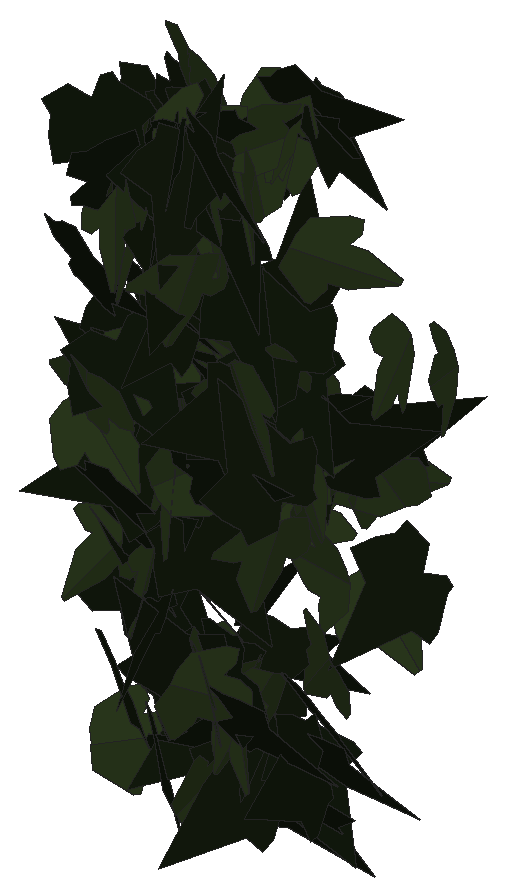
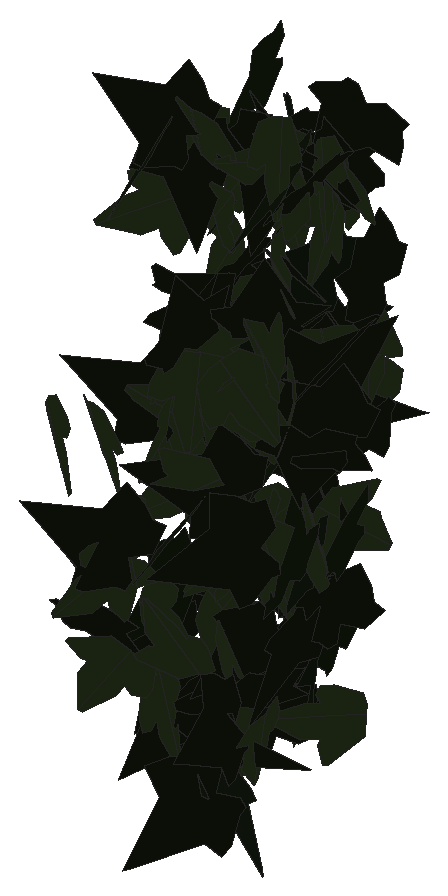
# SketchUp Ruby script. Lengths in inches.
U = 1.inch
M = Sketchup.active_model
def pt(a) = Geom::Point3d.new(a.map { |v| v * U })
def face(e, loops, mat)
  f = e.add_face(loops[0].map { |a| pt(a) })
  loops[1..].each { |l| e.add_face(l.map { |a| pt(a) }).erase! }
  f.material = f.back_material = mat if mat
  f
end
# faces: each face lists its corners as indices into pts; further lists are holes
def faces(e, pts, list, mat = nil) = list.each { |f| face(e, (f[0].is_a?(Array) ? f : [f]).map { |l| l.map { |i| pts[i] } }, mat) }
# xy, xz, yz: faces in a plane at the given z, y or x. An outline is a flat list of corners, or four numbers for a rectangle; further outlines are holes
def ring(l) = l.size == 4 ? [[l[0], l[1]], [l[2], l[1]], [l[2], l[3]], [l[0], l[3]]] : l.each_slice(2).to_a
def flat(e, list, mat, &to3) = list.each { |f| face(e, (f[0].is_a?(Array) ? f : [f]).map { |l| ring(l).map { |u, v| to3.(u, v) } }, mat) }
def xy(e, z, list, mat = nil) = flat(e, list, mat) { |x, y| [x, y, z] }
def xz(e, y, list, mat = nil) = flat(e, list, mat) { |x, z| [x, y, z] }
def yz(e, x, list, mat = nil) = flat(e, list, mat) { |y, z| [x, y, z] }
def lines(e, pts, list) = list.each { |a, b| e.add_line(pt(pts[a]), pt(pts[b])) }
# prism: a flat outline (further loops are holes) pulled along v
def prism(e, loops, v, mat = nil)
  f = face(e, loops, mat); d = Geom::Vector3d.new(v.map { |x| x * U })
  f.pushpull(f.normal.samedirection?(d) ? d.length : -d.length)
end
def box(e, o, s, mat = nil) = prism(e, [[o, [o[0] + s[0], o[1], o[2]], [o[0] + s[0], o[1] + s[1], o[2]], [o[0], o[1] + s[1], o[2]]]], [0, 0, s[2]], mat)
def at(x, y, z, deg = 0) = Geom::Transformation.translation(pt([x, y, z])) * Geom::Transformation.rotation(ORIGIN, Z_AXIS, deg.degrees)
def axes(o, x, y, z) = Geom::Transformation.new([*x, 0, *y, 0, *z, 0, *pt(o).to_a, 1])
def part(name) = M.definitions.add(name)
# library, detail: a bought-in or finely detailed component or shape, given as its bounding box
def library(name, o, s) = part(name).tap { |d| box(d.entities, o, s) }
def detail(e, o, s) = box(e.add_group.entities, o, s)
def put(e, d, t, mat = nil) = e.add_instance(d, t).tap { |i| i.material = mat if mat }
def group(e, t, mat = nil) = e.add_group.tap { |g| g.transformation = t; g.material = mat if mat }.entities
root = M.entities
M.materials.add("efeu1").color = [18, 25, 13]
M.materials.add("efeu2").color = [43, 57, 29]
c1 = part("ivyleaf_9")
p = [[1.54,2.16,1.25],[1.36,2.04,1.19],[-0.21,0.99,0.68],[-0.71,1.11,0.82],[-0.85,0.86,0.67],[-0.8,0.17,0.21],
  [-0.9,-0.01,0.1],[-0.67,-0.16,-0.02],[-0.08,-0.08,-0.05],[-0.03,-0.6,-0.4],[0.65,-0.88,-0.66],[0.83,-0.6,-0.49],
  [1.29,-0.42,-0.43],[1.8125,-0.07,-0.26],[1.21,0.44,0.15]]
faces(c1.entities,p,[[0,1,2,3,4,5,6,7,8,9,10,11,12,13,14]],"efeu1")
c2 = part("ivyleaf_10")
p = [[0,0.5,-0.03],[-0.0625,2.02,-0.43],[-0.19,2.01,-0.46],[-0.54,1.05,-0.29],[-0.52,0.625,-0.18],[-0.83,0.76,-0.28],
  [-1.16,0.64,-0.33],[-1.15,0.33,-0.24],[-0.77,-0.39,0.02],[-0.3,-0.51,0.16],[0.04,-0.48,0.23],[-0.02,2.01,-0.4375],
  [-0.06,2.01,-0.43],[0.04,-0.49,0.23],[0.67,-0.49,0.14],[1.38,0.36,-0.2],[1.375,0.51,-0.24],[0.81,0.65,-0.19],
  [0.62,0.59,-0.15],[0.6,1.09,-0.28],[0.5,1.23,-0.31]]
faces(c2.entities,p,[[0,1,2,3,4,5,6,7,8,9,10],[11,12,0,13,14,15,16,17,18,19,20]],"efeu2")
put(root,c1,axes([35.11,223.37,217.44],[0.41887,-0.24066,-0.12894],[-0.10462,0.07663,-0.48289],[0.25219,0.43152,0.01384]))
put(root,c1,axes([35.23,224.11,218.95],[-0.24521,-0.33335,-0.28062],[0.17028,0.22309,-0.4138],[0.40109,-0.29851,0.00412]))
put(root,c1,axes([34.97,223.83,218.99],[0.11939,-0.07912,0.47905],[0.46236,-0.13208,-0.13704],[0.14823,0.47571,0.04163]))
put(root,c2,axes([35.53,223.26,217.38],[-0.13067,-0.26306,0.40463],[-0.05565,-0.40819,-0.28335],[0.4794,-0.11909,0.0774]))
put(root,c1,axes([35.2,223.61,216.17],[-0.13742,0.01876,0.48038],[0.47886,-0.03889,0.13851],[0.04256,0.49813,-0.00728]))
put(root,c1,axes([35.72,225.29,214.58],[-0.26797,0.41954,0.04669],[-0.02794,0.03755,-0.4978],[-0.4212,-0.2694,0.00332]))
put(root,c2,axes([35.38,223.7,216.95],[0.28986,-0.40739,-0.00394],[0.00449,-0.00164,0.49998],[-0.40739,-0.28988,0.00271]))
put(root,c1,axes([35.42,224,216.1875],[0.14476,-0.23263,-0.41824],[-0.21797,0.35696,-0.27398],[0.42607,0.26165,0.00194]))
put(root,c1,axes([35.08,222.9,220.77],[0.24977,-0.19631,0.38611],[0.29109,-0.25397,-0.31743],[0.32075,0.38335,-0.01258]))
put(root,c2,axes([35.42,224.85,215.12],[-0.04426,0.49201,-0.07725],[0.00837,-0.07681,-0.49399],[-0.49797,-0.04502,-0.00144]))
put(root,c1,axes([35.5,225.33,215.32],[0.06139,0.22899,0.44022],[0.13132,0.42027,-0.23692],[-0.47853,0.14471,-0.00854]))
put(root,c1,axes([35.3,223.6,219.8125],[0.06581,-0.4799,0.12394],[0.03016,-0.12092,-0.48422],[0.49473,0.07121,0.01303]))
put(root,c1,axes([35.33,225.94,214.64],[0.41277,0.24469,0.14052],[0.12007,0.07302,-0.47985],[-0.25535,0.42988,0.00152]))
put(root,c2,axes([35.27,223.34,214.64],[0.05743,-0.04345,-0.49479],[0.41152,0.28306,0.02291],[0.27812,-0.40986,0.06827]))
put(root,c2,axes([35.71,222.39,219.64],[-0.48065,0.03711,0.13265],[-0.13227,0.01008,-0.48208],[-0.03845,-0.49852,0.00013]))
put(root,c1,axes([35.8,223.35,219.15],[0.10877,0.02796,0.48722],[-0.48134,-0.07619,0.11183],[0.0805,-0.49337,0.01035]))
put(root,c2,axes([35.58,223.28,221.6875],[-0.42485,0.26195,-0.02976],[0.02473,-0.0166,-0.49911],[-0.26247,-0.42557,0.00115]))
put(root,c1,axes([35.42,223.96,222.47],[0.04736,-0.49619,0.03945],[0.01761,-0.03793,-0.49825],[0.49744,0.04858,0.01388]))
put(root,c1,axes([35.375,225.01,217.75],[0.28746,0.18449,0.36514],[0.3003,0.20791,-0.34146],[-0.27782,0.41562,0.00872]))
put(root,c1,axes([35.36,224.36,217.07],[0.37616,-0.19146,-0.26804],[0.24095,-0.11749,0.42206],[-0.22461,-0.4467,0.00388]))
put(root,c2,axes([35.82,224.03,223.04],[-0.43216,0.1415,0.20788],[-0.19349,0.07688,-0.45459],[-0.16062,-0.47336,-0.01169]))
put(root,c2,axes([35.72,223.19,222.4],[0.1112,-0.45507,-0.17477],[-0.02862,0.17286,-0.4683],[0.48664,0.11415,0.0124]))
put(root,c2,axes([35.69,224.3125,217.26],[0.08688,-0.47772,0.11932],[0.0325,-0.11533,-0.48543],[0.49132,0.0921,0.01101]))
put(root,c1,axes([36.13,225.24,214.84],[-0.36335,-0.01145,0.34328],[-0.34323,-0.00665,-0.36352],[0.01289,-0.49982,-0.00303]))
put(root,c2,axes([36.09,223.96,218.9],[0.05965,0.00155,-0.49643],[-0.47281,-0.15222,-0.05728],[-0.1513,0.47626,-0.0167]))
put(root,c2,axes([35.44,224.55,220.08],[-0.10964,0.0224,0.48732],[0.46723,-0.1388,0.1115],[0.14028,0.47982,0.0095]))
put(root,c1,axes([35.61,223.96,222.66],[0.38029,-0.24282,-0.21546],[-0.14822,0.16536,-0.44798],[0.28881,0.40459,0.05379]))
put(root,c1,axes([35.53,222.66,222.99],[-0.15015,-0.16353,-0.44801],[0.32706,0.30654,-0.22151],[0.34711,-0.35957,0.01491]))
put(root,c2,axes([35.61,224.03,219.35],[-0.15125,0.28226,-0.38399],[0.17892,-0.33977,-0.32023],[-0.44171,-0.23428,0.00178]))
put(root,c1,axes([35.56,223.13,215.52],[0.02902,-0.19959,0.45752],[0.15002,-0.43361,-0.19868],[0.47608,0.1488,0.03472]))
put(root,c2,axes([35.77,223.15,219.76],[0.38168,0.31827,-0.055],[-0.04252,-0.0349,-0.49697],[-0.32018,0.38404,0.00043]))
put(root,c2,axes([36.07,224.64,219.76],[-0.30192,-0.25974,0.30229],[-0.21257,-0.21584,-0.39777],[0.33713,-0.36871,0.01991]))
put(root,c1,axes([36.11,222.93,218.58],[-0.07723,-0.19879,-0.45224],[-0.10899,-0.43959,0.21185],[-0.48183,0.1313,0.02457]))
put(root,c2,axes([35.61,222.46,219.2],[0.33561,0.22296,0.29606],[0.25085,0.15738,-0.40287],[-0.27284,0.41895,-0.00622]))
put(root,c1,axes([35.74,222.33,218.55],[0.48148,0.07307,-0.11331],[-0.11189,-0.01795,-0.48699],[-0.07524,0.49431,-0.00093]))
put(root,c1,axes([35.54,223.8,216.97],[0.39706,-0.2638,0.15084],[0.12924,-0.07802,-0.47666],[0.27503,0.41752,0.00623]))
put(root,c2,axes([35.68,226.01,216.47],[0.44446,-0.00098,-0.22903],[0.22785,0.05266,0.44194],[0.02325,-0.49722,0.04726]))
put(root,c2,axes([36.09,224.58,219.41],[0.26444,0.21311,-0.36695],[-0.32739,-0.17262,-0.33618],[-0.26998,0.41807,0.04824]))
put(root,c1,axes([35.67,222.48,222.15],[0.25324,0.125,0.41261],[0.36552,0.1915,-0.28235],[-0.22862,0.44464,0.00561]))
put(root,c2,axes([35.78,222.65,221.89],[0.42237,-0.1762,0.20138],[0.19446,-0.05637,-0.45717],[0.18381,0.46452,0.02091]))
put(root,c1,axes([35.82,222.74,220.02],[-0.03193,-0.31942,-0.38334],[0.119,0.36817,-0.31669],[0.48458,-0.11146,0.05251]))
put(root,c2,axes([36.0625,224.56,217.26],[0.01299,0.04959,0.49737],[-0.10661,0.48636,-0.0457],[-0.48833,-0.10487,0.02321]))
put(root,c1,axes([36.25,224.1875,214.95],[-0.32221,-0.2956,0.24249],[-0.17196,-0.17119,-0.43718],[0.34148,-0.36512,0.00865]))
put(root,c1,axes([36.37,223.55,222.48],[-0.4892,-0.03288,0.09797],[-0.09709,-0.01611,-0.49022],[0.0354,-0.49866,0.00938]))
put(root,c1,axes([35.72,223.11,220.66],[0.32158,-0.23998,0.29832],[0.25134,-0.16156,-0.40091],[0.28881,0.40781,0.01672]))
put(root,c1,axes([35.97,224.25,218.03],[-0.01879,-0.36522,0.34097],[0.03743,-0.34129,-0.36349],[0.49824,0.01187,0.04016]))
put(root,c1,axes([35.93,223.4,214.48],[0.01277,-0.11607,0.48617],[0.09594,-0.47672,-0.11633],[0.49054,0.09626,0.0101]))
put(root,c1,axes([36.26,223.74,220.06],[-0.41795,-0.16121,0.2221],[0.21248,0.06603,0.44777],[-0.1737,0.46867,0.01332]))
put(root,c1,axes([35.9,223.02,217.26],[-0.06107,0.09764,0.48656],[0.29406,-0.38777,0.11472],[0.39975,0.30017,-0.01007]))
put(root,c2,axes([36.25,222.51,221.72],[0.30026,-0.39695,-0.04767],[-0.02885,0.03794,-0.49772],[0.39876,0.30164,-0.00012]))
put(root,c1,axes([36.24,223.46,222.58],[0.30048,0.38408,-0.11043],[-0.07085,-0.08478,-0.48764],[-0.39331,0.3087,0.00347]))
put(root,c2,axes([36.17,222.82,217.55],[0.35041,-0.34361,0.09561],[0.06886,-0.06634,-0.49077],[0.34996,0.35711,0.00083]))
put(root,c2,axes([35.89,223.625,222.09],[-0.1257,0.03507,-0.48267],[0.42294,-0.23442,-0.12718],[-0.23521,-0.44025,0.02926]))
put(root,c1,axes([36.02,223.84,214.39],[0.45386,0.19835,0.06833],[-0.0676,-0.0159,0.49515],[0.1986,-0.4587,0.01239]))
put(root,c1,axes([36.45,223.08,220.55],[-0.4907,0.07951,-0.05378],[0.05327,-0.00747,-0.4971],[-0.07986,-0.49358,-0.00114]))
put(root,c1,axes([35.9,224.79,218.24],[0.18575,0.00341,0.46421],[0.459,0.07338,-0.1842],[-0.06938,0.49457,0.02413]))
put(root,c2,axes([36.15,223.57,220.875],[0.26451,-0.28956,0.31014],[0.20161,-0.23581,-0.39211],[0.37334,0.33249,-0.00799]))
put(root,c2,axes([36.07,223.44,222.36],[0.06505,0.03302,-0.49465],[0.34012,0.35999,0.06876],[0.36067,-0.34543,0.02438]))
put(root,c1,axes([36.08,225.88,217.97],[0.10408,-0.46346,0.15613],[0.04191,-0.15059,-0.47494],[0.48725,0.11194,0.0075]))
put(root,c1,axes([36.34,222.9,217.11],[-0.34358,0.12262,-0.34193],[0.30736,-0.15271,-0.3636],[-0.19361,-0.46005,0.02956]))
put(root,c2,axes([36.3,223.88,214.26],[0.00266,0.14559,0.47833],[0.01517,0.47809,-0.1456],[-0.49976,0.01529,-0.00187]))
put(root,c1,axes([36.3,223.12,222.6],[-0.26525,0.05667,-0.42004],[0.39923,-0.13298,-0.27005],[-0.14232,-0.47865,0.02529]))
put(root,c1,axes([36.57,222.92,216.03],[0.26558,-0.04971,0.42071],[-0.4055,0.11391,0.26943],[-0.12263,-0.48431,0.02019]))
put(root,c1,axes([36.2,223.63,215.72],[-0.02949,-0.14551,-0.47745],[0.12947,0.45968,-0.1481],[0.48205,-0.13236,0.01056]))
put(root,c2,axes([36.81,225.16,215.31],[-0.31378,0.10324,0.37534],[-0.36425,0.09222,-0.32988],[-0.13735,-0.48045,0.01734]))
put(root,c1,axes([36.54,222.86,222.04],[-0.37488,0.30609,0.12561],[0.09597,-0.08107,0.48396],[0.31663,0.38696,0.00203]))
put(root,c2,axes([36.26,224.99,218.33],[0.13189,0.16552,0.453],[0.27203,0.36227,-0.21156],[-0.39826,0.30226,0.00551]))
put(root,c2,axes([36.86,225.18,216.42],[0.082,-0.04456,-0.49121],[-0.40511,0.27796,-0.09284],[0.28135,0.41322,0.00948]))
put(root,c2,axes([36.52,223.21,214.36],[0.05428,-0.2838,0.40806],[-0.02389,0.40852,0.2873],[-0.49647,-0.05069,0.0308]))
put(root,c2,axes([36.76,224.09,221.65],[0.35124,-0.08107,0.34649],[-0.32948,0.10983,0.3597],[-0.13444,-0.481,0.02373]))
put(root,c1,axes([36.45,222.91,221.26],[-0.00194,-0.41269,0.28228],[0.0149,-0.2822,-0.41248],[0.49977,0.00681,0.01339]))
put(root,c2,axes([36.67,223.89,215.65],[0.11441,-0.46423,0.14627],[0.03267,-0.1426,-0.47812],[0.48564,0.11896,-0.0023]))
put(root,c1,axes([36.61,223.11,222.39],[-0.16349,-0.47012,0.04754],[-0.01569,-0.04487,-0.49774],[0.47226,-0.16424,-0.00008]))
put(root,c1,axes([36.99,223.76,218.28],[-0.28282,0.37753,0.16578],[-0.10541,0.12815,-0.47166],[-0.39862,-0.30175,0.00711]))
put(root,c2,axes([36.47,222.8,218.71],[0.30008,-0.22495,0.33068],[0.27002,-0.19102,-0.37497],[0.29503,0.40362,0.00684]))
put(root,c1,axes([36.79,224.66,220.02],[-0.16671,-0.28768,0.37343],[0.22334,0.30061,0.33129],[-0.41512,0.27726,0.02826]))
put(root,c1,axes([36.36,223.78,219.17],[0.31325,-0.2476,0.30095],[0.24595,-0.17392,-0.39908],[0.3023,0.39806,0.01283]))
put(root,c2,axes([36.86,224.36,219.45],[-0.47399,-0.15791,0.02006],[-0.01831,-0.00852,-0.49959],[0.15812,-0.47433,0.00229]))
put(root,c2,axes([36.9375,222.57,221.42],[-0.20033,-0.44711,0.09983],[-0.03568,-0.0934,-0.4899],[0.45672,-0.20341,0.00552]))
put(root,c2,axes([36.6,223.1,222.14],[0.41104,-0.08213,0.27258],[0.27443,-0.01299,-0.41775],[0.07571,0.49304,0.0344]))
put(root,c2,axes([36.72,222.61,218.71],[-0.06295,-0.15933,0.46974],[0.16223,0.44085,0.17127],[-0.46874,0.17397,-0.0038]))
put(root,c2,axes([37.16,224.13,222.51],[0.09809,0.14437,-0.46855],[-0.40584,-0.24419,-0.1602],[-0.27509,0.41174,0.06928]))
put(root,c2,axes([36.62,223.78,221.97],[0.29502,-0.11973,0.38553],[0.35965,-0.13893,-0.31836],[0.18335,0.46515,0.00415]))
put(root,c1,axes([37.14,223.49,214.6875],[-0.48961,-0.09045,0.04587],[-0.04442,-0.01199,-0.49788],[0.09116,-0.4916,0.00371]))
put(root,c2,axes([36.93,223.98,218.44],[0.27383,-0.41512,0.05192],[0.03257,-0.04071,-0.49727],[0.41708,0.27571,0.00474]))
put(root,c1,axes([37.3,222.98,216.34],[0.00316,0.04568,-0.4979],[-0.47487,-0.15557,-0.01729],[-0.15649,0.47298,0.0424]))
put(root,c2,axes([37.15,225.86,217.28],[-0.40937,-0.1467,-0.24678],[-0.23076,-0.08753,0.43484],[-0.17078,0.46991,0.00396]))
put(root,c2,axes([37.3,223.75,219.59],[-0.26177,0.00512,-0.42597],[-0.42172,-0.07386,0.25826],[-0.06028,0.49449,0.04299]))
put(root,c2,axes([36.87,225.94,217.37],[-0.11384,-0.18612,-0.44989],[0.22488,0.38968,-0.21811],[0.43182,-0.25201,-0.00501]))
put(root,c1,axes([36.66,226.04,217.66],[0.09202,-0.06429,0.48724],[0.4882,0.06895,-0.0831],[-0.05651,0.49103,0.07546]))
put(root,c1,axes([37.1,224.07,222.64],[0.26842,0.33894,-0.25114],[-0.16592,-0.18886,-0.43221],[-0.38784,0.31536,0.01108]))
put(root,c2,axes([37.0625,223.62,215.74],[-0.03065,-0.42349,0.26404],[0.00296,-0.26469,-0.42418],[0.49905,-0.02444,0.01873]))
put(root,c2,axes([36.96,224.19,222.92],[0.48796,-0.1036,0.0341],[0.03369,-0.00553,-0.49883],[0.10374,0.48912,0.00159]))
put(root,c1,axes([36.85,223.61,220.68],[0.13655,-0.47131,-0.09603],[-0.02746,0.09202,-0.49069],[0.48021,0.13928,-0.00075]))
put(root,c2,axes([37.07,223.18,219.77],[0.06466,-0.39312,0.30212],[0.03274,-0.30063,-0.39818],[0.49472,0.07128,-0.01314]))
put(root,c1,axes([36.83,223.43,221.72],[0.18478,-0.45024,0.11463],[0.03864,-0.10804,-0.48666],[0.46299,0.18871,-0.00513]))
put(root,c2,axes([37.06,222.61,216.58],[-0.31497,0.38708,-0.03102],[0.01782,-0.02548,-0.49903],[-0.38791,-0.31547,0.00225]))
put(root,c1,axes([36.87,222.875,217.97],[-0.13422,-0.18504,-0.44469],[0.24357,0.37217,-0.22838],[0.41552,-0.27794,-0.00976]))
put(root,c2,axes([36.88,225.8125,215.96],[0.34065,0.2253,0.28844],[0.24003,0.15994,-0.40842],[-0.2763,0.41673,0.00081]))
put(root,c2,axes([36.86,223.37,215.61],[0.29226,-0.1559,0.37453],[0.35566,-0.12359,-0.32898],[0.19516,0.45871,0.03865]))
put(root,c1,axes([37.03,222.62,223.08],[0.41448,-0.20987,-0.18482],[-0.16207,0.08902,-0.46455],[0.2279,0.445,0.00577]))
put(root,c1,axes([37.57,223.65,219.98],[-0.47833,-0.10065,-0.10524],[-0.10218,-0.02546,0.48879],[-0.10375,0.4891,0.00378]))
put(root,c1,axes([37.09,222.96,219.64],[0.16622,-0.44477,-0.15667],[-0.06607,0.14252,-0.47468],[0.46691,0.17851,-0.0114]))
put(root,c2,axes([37.37,225.69,219.2],[0.38976,-0.28566,-0.12839],[-0.0996,0.08126,-0.48319],[0.29692,0.40224,0.00644]))
put(root,c2,axes([37.17,222.27,216.43],[-0.1726,-0.19024,-0.42898],[0.29074,0.31542,-0.25686],[0.36835,-0.33811,0.00174]))
put(root,c1,axes([37.58,225.77,216.43],[-0.4913,-0.0928,0.00399],[-0.00379,-0.00146,-0.49998],[0.09281,-0.49131,0.00074]))
put(root,c2,axes([37.11,223.98,218.4375],[-0.18305,-0.12607,0.44788],[0.36664,0.25725,0.22226],[-0.28647,0.4098,-0.00174]))
put(root,c1,axes([37.22,223.71,219.9],[-0.06922,-0.3221,-0.37611],[0.09504,0.36407,-0.32928],[0.48598,-0.11707,0.01082]))
put(root,c1,axes([37.02,222.6,218.85],[0.15993,-0.08765,0.46555],[0.40485,-0.22988,-0.18235],[0.24601,0.43529,-0.00256]))
put(root,c1,axes([37.52,222.88,219.69],[0.06231,-0.32194,-0.37746],[0.07077,-0.37076,0.32791],[-0.49103,-0.09429,-0.00064]))
put(root,c2,axes([37.49,223.95,218.36],[0.0014,-0.20811,-0.45463],[0.03154,0.45376,-0.20761],[0.499,-0.0281,0.0144]))
put(root,c1,axes([37.3,223.9,214.94],[-0.02851,-0.33497,-0.37011],[0.10238,0.35891,-0.33272],[0.48857,-0.09476,0.04813]))
put(root,c1,axes([37.39,224.3,222.78],[0.3421,-0.23781,-0.27643],[-0.19802,0.19713,-0.41464],[0.3062,0.39318,0.0407]))
put(root,c1,axes([37.33,223.73,214.38],[0.48211,0.13158,0.01613],[0.01485,0.00683,-0.49973],[-0.13173,0.48233,0.00268]))
put(root,c1,axes([37.14,224.27,222.75],[0.15485,-0.14435,0.45297],[0.43511,-0.14895,-0.19621],[0.19159,0.45495,0.07949]))
put(root,c1,axes([37.3,222.75,215.92],[0.44107,-0.09107,0.21718],[0.21323,-0.04129,-0.45036],[0.09996,0.4899,0.00241]))
put(root,c2,axes([37.91,225.87,219.08],[0.23161,-0.23083,-0.37825],[-0.22568,0.30586,-0.32484],[0.38135,0.3212,0.03749]))
put(root,c2,axes([37.71,223.58,218.9],[-0.13443,0.47887,0.0511],[-0.01663,0.04841,-0.49737],[-0.4813,-0.13543,0.00291]))
put(root,c2,axes([37.72,222.57,220.27],[-0.35546,0.24743,-0.24986],[0.18279,-0.17349,-0.43184],[-0.3004,-0.39834,0.03288]))
put(root,c2,axes([37.95,222.79,218.36],[-0.17402,-0.45968,0.09173],[-0.02869,-0.08722,-0.4915],[0.46786,-0.17633,0.00398]))
put(root,c1,axes([37.51,223.875,215.05],[0.4447,-0.08368,0.21269],[0.21297,-0.01719,-0.45205],[0.08297,0.49265,0.02036]))
put(root,c1,axes([37.7,223.59,215.93],[0.47769,-0.1321,-0.06608],[-0.06412,0.01605,-0.49561],[0.13306,0.48197,-0.00161]))
put(root,c1,axes([37.55,224.125,218.6],[0.09321,-0.01164,0.4911],[0.48926,-0.04259,-0.09387],[0.04402,0.49805,0.00345]))
put(root,c1,axes([38.13,222.63,218.98],[-0.31427,-0.3769,0.09582],[0.06868,0.06747,0.49064],[-0.38278,0.32155,0.00937]))
put(root,c1,axes([37.93,223.5,215.09],[-0.06483,-0.23883,0.43446],[-0.13633,-0.41268,-0.2472],[0.47667,-0.15051,-0.01161]))
put(root,c2,axes([37.7,223.77,221.4],[-0.19325,-0.07579,-0.45487],[0.41862,0.17802,-0.20751],[0.19341,-0.46105,-0.00536]))
